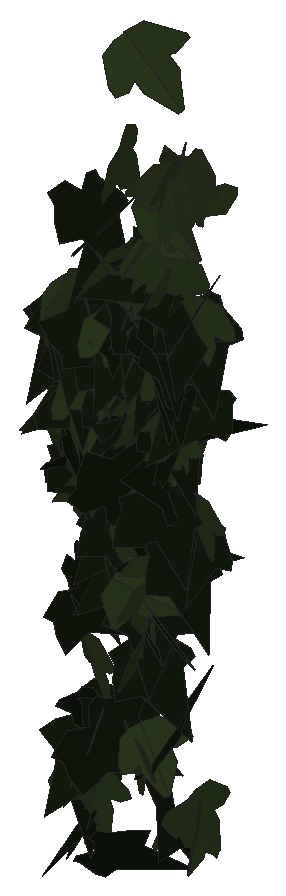
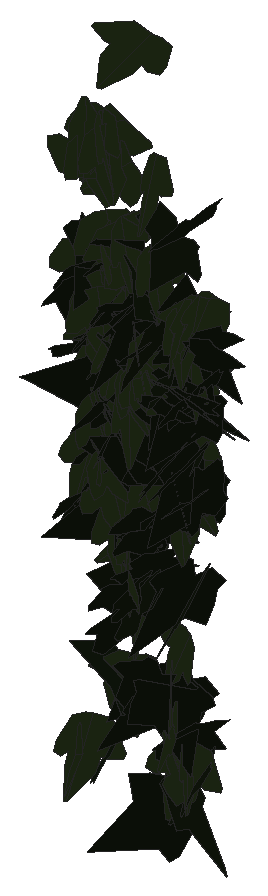
# SketchUp Ruby script. Lengths in inches.
U = 1.inch
M = Sketchup.active_model
def pt(a) = Geom::Point3d.new(a.map { |v| v * U })
def face(e, loops, mat)
  f = e.add_face(loops[0].map { |a| pt(a) })
  loops[1..].each { |l| e.add_face(l.map { |a| pt(a) }).erase! }
  f.material = f.back_material = mat if mat
  f
end
# faces: each face lists its corners as indices into pts; further lists are holes
def faces(e, pts, list, mat = nil) = list.each { |f| face(e, (f[0].is_a?(Array) ? f : [f]).map { |l| l.map { |i| pts[i] } }, mat) }
# xy, xz, yz: faces in a plane at the given z, y or x. An outline is a flat list of corners, or four numbers for a rectangle; further outlines are holes
def ring(l) = l.size == 4 ? [[l[0], l[1]], [l[2], l[1]], [l[2], l[3]], [l[0], l[3]]] : l.each_slice(2).to_a
def flat(e, list, mat, &to3) = list.each { |f| face(e, (f[0].is_a?(Array) ? f : [f]).map { |l| ring(l).map { |u, v| to3.(u, v) } }, mat) }
def xy(e, z, list, mat = nil) = flat(e, list, mat) { |x, y| [x, y, z] }
def xz(e, y, list, mat = nil) = flat(e, list, mat) { |x, z| [x, y, z] }
def yz(e, x, list, mat = nil) = flat(e, list, mat) { |y, z| [x, y, z] }
def lines(e, pts, list) = list.each { |a, b| e.add_line(pt(pts[a]), pt(pts[b])) }
# prism: a flat outline (further loops are holes) pulled along v
def prism(e, loops, v, mat = nil)
  f = face(e, loops, mat); d = Geom::Vector3d.new(v.map { |x| x * U })
  f.pushpull(f.normal.samedirection?(d) ? d.length : -d.length)
end
def box(e, o, s, mat = nil) = prism(e, [[o, [o[0] + s[0], o[1], o[2]], [o[0] + s[0], o[1] + s[1], o[2]], [o[0], o[1] + s[1], o[2]]]], [0, 0, s[2]], mat)
def at(x, y, z, deg = 0) = Geom::Transformation.translation(pt([x, y, z])) * Geom::Transformation.rotation(ORIGIN, Z_AXIS, deg.degrees)
def axes(o, x, y, z) = Geom::Transformation.new([*x, 0, *y, 0, *z, 0, *pt(o).to_a, 1])
def part(name) = M.definitions.add(name)
# library, detail: a bought-in or finely detailed component or shape, given as its bounding box
def library(name, o, s) = part(name).tap { |d| box(d.entities, o, s) }
def detail(e, o, s) = box(e.add_group.entities, o, s)
def put(e, d, t, mat = nil) = e.add_instance(d, t).tap { |i| i.material = mat if mat }
def group(e, t, mat = nil) = e.add_group.tap { |g| g.transformation = t; g.material = mat if mat }.entities
root = M.entities
M.materials.add("efeu1").color = [18, 25, 13]
M.materials.add("efeu2").color = [43, 57, 29]
c1 = part("ivyleaf_9")
p = [[1.54,2.16,1.25],[1.36,2.04,1.19],[-0.21,0.99,0.68],[-0.71,1.11,0.82],[-0.85,0.86,0.67],[-0.8,0.17,0.21],
  [-0.9,-0.01,0.1],[-0.67,-0.16,-0.02],[-0.08,-0.08,-0.05],[-0.03,-0.6,-0.4],[0.65,-0.88,-0.66],[0.83,-0.6,-0.49],
  [1.29,-0.42,-0.43],[1.8125,-0.07,-0.26],[1.21,0.44,0.15]]
faces(c1.entities,p,[[0,1,2,3,4,5,6,7,8,9,10,11,12,13,14]],"efeu1")
c2 = part("ivyleaf_10")
p = [[0,0.5,-0.03],[-0.0625,2.02,-0.43],[-0.19,2.01,-0.46],[-0.54,1.05,-0.29],[-0.52,0.625,-0.18],[-0.83,0.76,-0.28],
  [-1.16,0.64,-0.33],[-1.15,0.33,-0.24],[-0.77,-0.39,0.02],[-0.3,-0.51,0.16],[0.04,-0.48,0.23],[-0.02,2.01,-0.4375],
  [-0.06,2.01,-0.43],[0.04,-0.49,0.23],[0.67,-0.49,0.14],[1.38,0.36,-0.2],[1.375,0.51,-0.24],[0.81,0.65,-0.19],
  [0.62,0.59,-0.15],[0.6,1.09,-0.28],[0.5,1.23,-0.31]]
faces(c2.entities,p,[[0,1,2,3,4,5,6,7,8,9,10],[11,12,0,13,14,15,16,17,18,19,20]],"efeu2")
put(root,c1,axes([533.84,134.95,193.96],[-0.16592,-0.62665,-0.45932],[0.10386,0.44757,-0.64814],[0.76999,-0.19541,-0.01155]))
put(root,c2,axes([533.1,134.63,191.76],[-0.18659,-0.42334,-0.62517],[0.57228,0.34075,-0.40155],[0.49248,-0.55636,0.22975]))
put(root,c2,axes([534.55,135.05,202.51],[-0.46736,-0.64643,0.18683],[-0.07545,-0.17569,-0.79664],[0.66864,-0.47166,0.04069]))
put(root,c2,axes([533.58,134.75,187.75],[0.40332,0.56558,0.24405],[0.1589,0.18631,-0.69437],[-0.59514,0.43303,-0.02001]))
put(root,c1,axes([532.63,134.49,193.875],[-0.1427,-0.17651,0.84402],[0.72497,0.4386,0.2143],[-0.46683,0.73509,0.0748]))
put(root,c2,axes([530.71,135.16,194.8],[-0.30059,0.19641,-0.75857],[0.60278,-0.46117,-0.35826],[-0.50067,-0.67314,0.02411]))
put(root,c2,axes([533.76,134.85,202.09],[0.51875,-0.04959,0.64712],[0.63525,0.20854,-0.49325],[-0.13298,0.80273,0.16812]))
put(root,c2,axes([534.21,134.89,196.51],[-0.68223,-0.41201,-0.00439],[0.00274,0.00396,-0.79699],[0.41203,-0.68223,-0.00197]))
put(root,c1,axes([531.37,134.625,195.06],[0.57411,-0.19969,-0.53388],[-0.46694,0.26982,-0.60305],[0.32691,0.73609,0.07622]))
put(root,c1,axes([533.58,135.35,198.11],[0.13758,-0.75271,0.21451],[0.10161,-0.19877,-0.76268],[0.77605,0.15947,0.06184]))
put(root,c2,axes([533.23,134.77,187.43],[-0.61959,0.35525,0.16784],[-0.16104,0.05627,-0.71356],[-0.35838,-0.63945,0.03046]))
put(root,c2,axes([532.5,134.86,198.36],[0.66095,0.3724,0.21897],[0.16704,0.1488,-0.75726],[-0.3984,0.6802,0.04577]))
put(root,c1,axes([534.33,135.1,192.72],[0.17347,-0.76248,-0.20975],[-0.0096,0.21269,-0.78111],[0.79075,0.16985,0.03653]))
put(root,c1,axes([531.48,135.49,186.59],[-0.39582,-0.61012,0.23934],[-0.07368,-0.2364,-0.7245],[0.65123,-0.39758,0.0635]))
put(root,c1,axes([532.14,134.83,197.82],[-0.63503,-0.42973,0.35723],[0.32377,0.15782,0.76539],[-0.45548,0.71132,0.046]))
put(root,c2,axes([534.24,135.01,203.12],[0.22032,-0.80028,-0.06678],[-0.01386,0.06545,-0.83005],[0.80295,0.22072,0.00399]))
put(root,c2,axes([534.125,135.05,200.32],[-0.64051,-0.45772,0.15302],[-0.09081,-0.13544,-0.78522],[0.474,-0.64445,0.05634]))
put(root,c1,axes([531.2,135.29,197.93],[-0.75961,-0.27683,-0.11932],[0.10828,0.05132,-0.8084],[0.28133,-0.76721,-0.01102]))
put(root,c2,axes([531.57,134.96,196.35],[0.34137,0.71991,-0.0217],[-0.00719,-0.02061,-0.79674],[-0.7202,0.34144,-0.00234]))
put(root,c1,axes([533.98,135.39,197.95],[0.13306,-0.79394,0.12439],[-0.00172,-0.12636,-0.8047],[0.80362,0.13118,-0.02231]))
put(root,c1,axes([532.14,135.25,196.45],[-0.81999,-0.00074,0.27979],[-0.27979,0.00771,-0.81995],[-0.00179,-0.86637,-0.00754]))
put(root,c2,axes([533.41,134.98,191.61],[0.03767,-0.74397,-0.14396],[-0.0036,0.14396,-0.74491],[0.75776,0.03767,0.00362]))
put(root,c2,axes([533.67,135.02,199.05],[-0.80206,-0.11083,0.10074],[-0.08251,-0.13107,-0.80109],[0.125,-0.79766,0.11763]))
put(root,c1,axes([531.24,135.35,198.1],[-0.31647,-0.71563,-0.13253],[0.05105,0.12233,-0.78248],[0.72601,-0.32055,-0.00274]))
put(root,c2,axes([533.07,135,199.59],[-0.6543,-0.46309,0.03838],[-0.03555,-0.0162,-0.80156],[0.46331,-0.65522,-0.0073]))
put(root,c2,axes([531.23,134.66,198.75],[-0.04867,-0.59501,-0.55283],[0.24229,0.51797,-0.57882],[0.77521,-0.19924,0.1462]))
put(root,c1,axes([533.71,135.63,194.3125],[-0.2466,-0.13898,0.76089],[-0.18699,-0.76422,-0.2002],[0.75053,-0.23607,0.20012]))
put(root,c1,axes([534.69,135.6,197.02],[-0.52563,-0.56705,0.21694],[-0.02156,-0.26933,-0.75623],[0.60674,-0.50081,0.16106]))
put(root,c1,axes([532.72,135.4,198.29],[-0.64504,-0.46675,-0.16169],[0.15465,0.06176,-0.79521],[0.46914,-0.66212,0.03981]))
put(root,c1,axes([533.83,135.49,200.02],[-0.69769,-0.06374,0.38908],[-0.33584,-0.31818,-0.65436],[0.20653,-0.73274,0.25029]))
put(root,c2,axes([533.9,135.25,199.98],[0.2862,-0.75883,0.13365],[0.07281,-0.11529,-0.81055],[0.76706,0.29407,0.02708]))
put(root,c1,axes([534.41,135.47,199.37],[-0.18346,-0.78927,0.02669],[-0.00748,-0.02566,-0.81031],[0.78968,-0.18361,-0.00147]))
put(root,c1,axes([533.71,135.5,198.39],[0.17171,-0.75603,0.22366],[0.04403,-0.21935,-0.77527],[0.78719,0.17718,-0.00542]))
put(root,c1,axes([531.46,135.08,201.39],[0.31522,-0.69824,-0.32345],[0.00014,0.34959,-0.75452],[0.76952,0.28596,0.13264]))
put(root,c2,axes([534.05,135.14,202.87],[-0.32805,-0.75834,0.01412],[-0.00416,-0.01359,-0.82625],[0.75846,-0.32808,0.00158]))
put(root,c1,axes([533.875,135.48,198.03],[-0.6926,-0.32698,-0.26214],[0.30707,-0.05135,-0.74726],[0.2852,-0.73876,0.16797]))
put(root,c1,axes([531,135.54,185.22],[0.19734,-0.60262,0.41738],[0.13128,-0.3962,-0.63411],[0.72119,0.23702,0.00122]))
put(root,c1,axes([532.15,134.57,187.58],[0.1151,-0.15435,-0.89731],[-0.02892,0.90337,-0.1591],[0.91002,0.04823,0.10843]))
put(root,c2,axes([533.03,135.11,193.22],[-0.68755,-0.05511,0.38302],[-0.37043,-0.1321,-0.68395],[0.11191,-0.77587,0.08924]))
put(root,c1,axes([533.79,135.2,197.21],[-0.66198,0.42777,-0.04278],[-0.04593,-0.14846,-0.77388],[-0.42745,-0.64653,0.14939]))
put(root,c2,axes([531.19,134.84,198.81],[0.36313,0.65044,0.29531],[0.03551,0.31443,-0.73622],[-0.71346,0.34671,0.11366]))
put(root,c2,axes([532.39,135.41,196.875],[-0.22167,-0.71925,0.27722],[0.08408,-0.3093,-0.73524],[0.76623,-0.17414,0.16088]))
put(root,c2,axes([531.83,134.96,196.71],[-0.60272,0.50627,0.13738],[-0.12829,0.06065,-0.78634],[-0.50865,-0.6152,0.03553]))
put(root,c1,axes([533.62,135.73,185.44],[0.03368,-0.50018,0.60049],[0.05559,-0.59799,-0.50122],[0.77954,0.06425,0.0098]))
put(root,c2,axes([531.52,135.06,196.86],[-0.72153,0.24589,0.17205],[-0.19184,-0.03337,-0.75681],[-0.23078,-0.74101,0.09117]))
put(root,c2,axes([534.47,135.04,203.21],[-0.79112,0.17971,-0.03596],[0.03633,-0.00237,-0.81125],[-0.17963,-0.79193,-0.00573]))
put(root,c2,axes([533.54,135.26,200.47],[0.39155,0.66223,-0.25685],[-0.22739,-0.16099,-0.76171],[-0.67291,0.43973,0.10795]))
put(root,c2,axes([531.54,135.07,185.85],[-0.83355,-0.12212,-0.11742],[0.11619,0.01695,-0.84245],[0.12329,-0.84161,0.00007]))
put(root,c1,axes([531.68,135.18,184.96],[-0.58553,0.59707,-0.21516],[0.14057,-0.16346,-0.83615],[-0.61889,-0.60202,0.01364]))
put(root,c2,axes([533.13,134.91,205.9375],[0.52377,0.47337,0.55455],[0.40242,0.3817,-0.70591],[-0.608,0.66043,0.0105]))
put(root,c2,axes([533.1875,134.99,189.97],[0.15695,-0.66236,-0.39426],[-0.07468,0.3874,-0.68055],[0.7672,0.17321,0.01441]))
put(root,c1,axes([531.59,135.59,196.4375],[-0.76138,-0.19307,0.15907],[-0.13583,-0.10885,-0.78229],[0.21007,-0.77017,0.07069]))
put(root,c1,axes([533.46,135.69,197.37],[0.13564,-0.70848,0.34338],[0.07348,-0.33552,-0.7213],[0.78387,0.15404,0.0082]))
put(root,c1,axes([531.65,134.91,197.01],[0.69236,0.31292,-0.17973],[-0.1589,-0.08477,-0.7597],[-0.324,0.71027,-0.01149]))
put(root,c1,axes([533.12,135.625,198.68],[-0.34448,-0.72407,-0.02238],[0.01031,0.01988,-0.80183],[0.72434,-0.34463,0.00077]))
put(root,c2,axes([534.65,135.35,202.18],[-0.64248,-0.49641,-0.04392],[-0.03738,-0.02344,0.8119],[-0.49695,0.64355,-0.0043]))
put(root,c1,axes([533.93,135.34,195.5625],[-0.68086,0.33892,-0.24015],[0.21236,-0.11228,-0.76053],[-0.35699,-0.71319,0.00561]))
put(root,c1,axes([530.98,135.6,196.75],[0.03615,-0.7984,0.06051],[0.00888,-0.06017,-0.7992],[0.80064,0.03672,0.00613]))
put(root,c2,axes([533.51,135.2,192.21],[-0.39062,-0.68014,-0.06591],[0.027,0.06049,-0.7843],[0.68279,-0.3915,-0.00669]))
put(root,c1,axes([532.9,135.35,198.59],[0.28315,-0.72603,-0.20516],[-0.03004,0.2081,-0.77793],[0.75386,0.28099,0.04605]))
put(root,c2,axes([532.28,135.42,197.72],[-0.42013,-0.63714,0.21631],[-0.06227,-0.2171,-0.76042],[0.66997,-0.41972,0.06496]))
put(root,c2,axes([534.72,135.28,199.36],[-0.81575,-0.02654,-0.01615],[0.02151,-0.17598,-0.79686],[0.02242,-0.79671,0.17655]))
put(root,c2,axes([532.41,135.3,200.01],[-0.02902,-0.81791,-0.02892],[0.00048,0.02892,-0.81843],[0.81842,-0.02902,-0.00054]))
put(root,c1,axes([532.15,135.25,197.62],[0.11647,-0.66884,-0.43019],[0.10154,0.44373,-0.6624],[0.78873,0.04164,0.1488]))
put(root,c2,axes([534.01,135.28,198.74],[-0.59541,-0.53303,0.03518],[-0.00742,-0.04443,-0.79865],[0.53413,-0.59479,0.02813]))
put(root,c2,axes([531.4,135.18,186.09],[0.18111,-0.70138,-0.23666],[0.00765,0.2454,-0.72143],[0.74019,0.16907,0.06536]))
put(root,c1,axes([533.87,134.74,187.29],[-0.42501,0.76807,-0.09642],[-0.05251,0.08114,0.87779],[0.77231,0.42819,0.00662]))
put(root,c2,axes([533.65,135.62,193.99],[-0.20431,-0.64905,0.38443],[-0.03336,-0.39011,-0.67638],[0.75361,-0.19323,0.07427]))
put(root,c1,axes([534.84,134.65,199.16],[-0.0015,0.58299,0.5786],[0.00072,0.5786,-0.58299],[-0.82137,-0.00056,-0.00157]))
put(root,c2,axes([531.52,135.29,189.25],[-0.60517,0.36773,-0.23142],[0.17428,-0.15802,-0.70687],[-0.398,-0.62835,0.04233]))
put(root,c2,axes([533.02,135.51,196.48],[0.04216,-0.76807,0.17268],[-0.00077,-0.17297,-0.76916],[0.78724,0.04097,-0.01]))
put(root,c2,axes([534.0625,135.17,197.68],[0.3737,0.69499,0.06481],[-0.08724,0.11944,-0.77781],[-0.69253,0.35998,0.13295]))
put(root,c2,axes([533.73,135.42,193.22],[-0.52883,-0.53696,0.20001],[-0.1249,-0.15761,-0.75336],[0.55922,-0.54298,0.02089]))
put(root,c2,axes([531.47,135.04,193.67],[0.29315,-0.06457,-0.73666],[-0.58044,0.47088,-0.27226],[0.45817,0.63786,0.12641]))
put(root,c2,axes([532.92,135.3125,197.77],[0.33957,-0.71193,-0.17092],[-0.04585,0.16736,-0.7882],[0.73072,0.34134,0.02997]))
put(root,c1,axes([532.73,135.6,190.74],[0.49296,-0.46005,0.45299],[0.32039,-0.32051,-0.67415],[0.56053,0.58778,-0.01306]))
put(root,c1,axes([531.54,134.875,190.9375],[0.0862,-0.2132,-0.83177],[-0.22329,0.80162,-0.22862],[0.82912,0.23805,0.02491]))
put(root,c2,axes([533.27,135.41,200.59],[0.08287,-0.79862,-0.0637],[-0.00316,0.06371,-0.8029],[0.80115,0.08286,0.00342]))
put(root,c1,axes([531.53,135.67,197.35],[0.43106,-0.60047,0.29196],[0.15014,-0.25145,-0.73882],[0.65059,0.45588,-0.02294]))
put(root,c1,axes([531.18,135,196.37],[0.68529,0.36969,0.0047],[0.00342,0.00355,-0.77865],[-0.3697,0.6853,0.0015]))
put(root,c2,axes([533.58,135.31,197.13],[-0.14292,-0.74798,-0.20845],[0.20713,0.16754,-0.74322],[0.74834,-0.18923,0.16591]))
put(root,c1,axes([533.13,135.375,189.61],[0.13694,-0.65932,-0.42332],[0.05373,0.43662,-0.66267],[0.78167,0.08549,0.11971]))
put(root,c1,axes([534.48,135.6,198.93],[-0.0165,-0.76827,-0.23708],[0.01297,0.23685,-0.76841],[0.80391,-0.01958,0.00753]))
put(root,c2,axes([531.99,135.04,187.86],[0.12348,-0.41131,-0.65224],[-0.21939,0.61451,-0.42905],[0.73923,0.25108,-0.01838]))
put(root,c1,axes([531.82,135.375,187.84],[0.31205,0.47796,-0.50456],[-0.27493,-0.42307,-0.57081],[-0.63831,0.41588,-0.00081]))
put(root,c2,axes([531.45,135.4375,198.62],[0.01819,-0.80368,-0.13874],[0.029,0.13933,-0.80326],[0.81505,0.01298,0.03168]))
put(root,c1,axes([532.03,134.83,200.65],[0.18016,0.59753,0.49537],[-0.06744,0.51866,-0.6011],[-0.77323,0.09399,0.16785]))
put(root,c1,axes([532.02,134.97,184.09],[0.63363,0.29881,0.43485],[0.37735,0.21833,-0.69986],[-0.36877,0.73683,0.03103]))
put(root,c1,axes([531.5625,135.78,196.79],[-0.78567,0.00982,-0.0405],[0.03825,-0.13325,-0.77446],[-0.01652,-0.77534,0.13259]))
put(root,c1,axes([534.22,135.96,193],[-0.1481,-0.73998,0.15713],[0.00431,-0.16094,-0.75384],[0.75647,-0.14395,0.03506]))
put(root,c1,axes([532.26,135.56,192.86],[-0.12798,-0.65228,-0.39742],[0.05354,0.39431,-0.66441],[0.76194,-0.13728,-0.02007]))
put(root,c2,axes([532.33,135.74,196.99],[-0.4182,-0.61769,0.25766],[0.01408,-0.31188,-0.72482],[0.66913,-0.37949,0.17629]))
put(root,c1,axes([532.95,134.93,198.94],[-0.52428,0.35493,-0.59809],[-0.51385,0.30705,0.63265],[0.46866,0.7337,0.02457]))
put(root,c1,axes([532.96,135.81,190.68],[-0.16209,-0.7336,-0.13136],[0.00844,0.13261,-0.75103],[0.74522,-0.16107,-0.02006]))
put(root,c1,axes([533.38,134.88,192.48],[0.0592,0.32601,-0.80092],[0.07117,0.79824,0.33018],[0.8618,-0.08832,0.02775]))
put(root,c1,axes([530.47,135.86,193.76],[0.05316,-0.32791,0.71492],[0.51605,-0.52622,-0.27974],[0.59358,0.48686,0.17917]))
put(root,c2,axes([531.44,135.59,194.02],[0.41017,-0.64712,-0.09094],[-0.05793,0.07093,-0.76609],[0.65091,0.4141,-0.01088]))
put(root,c2,axes([531.4,135.53,185.39],[0.37193,-0.67752,0.04244],[-0.00023,0.04827,0.77255],[-0.67885,-0.37121,0.023]))
put(root,c1,axes([533.73,135.18,195.9],[0.48806,-0.02782,0.67419],[0.65889,0.19906,-0.46877],[-0.1455,0.80815,0.13867]))
put(root,c1,axes([532.37,136.12,191.53],[-0.47989,-0.4714,0.36402],[-0.15741,-0.35048,-0.66137],[0.57441,-0.48987,0.12289]))
put(root,c1,axes([532.28,135.87,196.1875],[-0.72832,-0.28605,-0.10521],[0.10288,0.02582,-0.78237],[0.2869,-0.73543,0.01345]))
put(root,c1,axes([532.13,136.08,192.71],[-0.47698,-0.5663,0.23462],[-0.10824,-0.2148,-0.73851],[0.60335,-0.48623,0.05299]))
put(root,c2,axes([534.34,136.03,185.45],[-0.07142,0.40787,-0.73489],[0.12034,-0.72497,-0.41406],[-0.83182,-0.1399,0.00319]))
put(root,c1,axes([531.55,135.67,194.75],[0.33761,-0.68678,-0.13482],[-0.02899,0.13583,-0.76454],[0.69928,0.3372,0.03339]))
put(root,c2,axes([533.95,135.77,195.4],[-0.10936,-0.76234,0.19115],[0.01716,-0.19527,-0.76892],[0.78576,-0.10183,0.0434]))
put(root,c1,axes([532.29,135.99,190.24],[0.22448,-0.51028,0.52232],[0.28366,-0.44259,-0.5543],[0.67287,0.35682,0.05942]))
put(root,c1,axes([530.875,135.8,193.8125],[0.13884,-0.74851,-0.12847],[0.11793,0.15027,-0.74803],[0.75024,0.1149,0.14136]))
put(root,c2,axes([533.61,135.67,195.51],[0.74811,-0.06392,0.21382],[0.21656,0.02721,-0.74956],[0.05392,0.77759,0.0438]))
put(root,c1,axes([532.08,135.5,188.21],[-0.11314,-0.32849,-0.69932],[0.38646,0.58795,-0.3387],[0.66903,-0.39517,0.07738]))
put(root,c1,axes([532.2,135.3125,198.71],[0.70697,0.02914,-0.36758],[-0.36854,0.08141,-0.70237],[0.01186,0.79265,0.08565]))
put(root,c1,axes([533.5,135.82,195.83],[0.16617,-0.76108,-0.1501],[-0.00411,0.15264,-0.77851],[0.77573,0.16384,0.02803]))
put(root,c2,axes([533.87,135.73,198.48],[-0.55071,-0.56145,0.13126],[-0.03853,-0.14527,-0.78303],[0.5753,-0.54718,0.07321]))
put(root,c2,axes([531.36,135.92,187.15],[-0.17333,0.57007,-0.49948],[0.05388,-0.50181,-0.59143],[-0.75602,-0.16646,0.07237]))
put(root,c1,axes([533.8,135.71,193.98],[-0.50523,0.11969,0.6047],[-0.58629,0.14819,-0.51918],[-0.19039,-0.77392,-0.00589]))
put(root,c2,axes([532.35,135.36,202.68],[0.12007,-0.66211,-0.46399],[0.05262,0.47448,-0.66347],[0.80678,0.06759,0.11233]))
put(root,c1,axes([530.91,135.55,191.09],[0.50601,-0.45467,-0.35821],[-0.26929,0.23625,-0.68026],[0.51237,0.57319,-0.00376]))
put(root,c2,axes([531.25,135.7,193.55],[-0.18863,-0.74442,-0.03497],[0.02005,0.03099,-0.76785],[0.74497,-0.18932,0.01181]))
put(root,c1,axes([531.02,135.93,194.77],[0.2189,-0.75711,-0.01729],[0.03612,0.02842,-0.78697],[0.75645,0.21773,0.04258]))
put(root,c1,axes([532.75,135.23,198.25],[0.10892,-0.2256,-0.76858],[-0.28046,0.71581,-0.24985],[0.7503,0.30032,0.01817]))
put(root,c2,axes([534.41,135.59,193.97],[-0.72361,0.2994,-0.01837],[0.01333,-0.01582,-0.78304],[-0.29966,-0.72367,0.00952]))
put(root,c2,axes([532.6,136.01,191.18],[0.38623,-0.32482,0.60183],[0.54425,-0.27254,-0.49638],[0.41412,0.66113,0.09106]))
put(root,c1,axes([532.03,136.09,192.73],[-0.19168,-0.75307,-0.01706],[0.00546,0.01621,-0.77708],[0.75325,-0.19175,0.00129]))
put(root,c2,axes([532.92,135.65,195.875],[-0.01768,-0.77943,-0.18772],[-0.0028,0.18783,-0.7796],[0.80172,-0.01654,-0.00687]))
put(root,c2,axes([531.41,135.36,198.87],[-0.33234,0.59061,0.40272],[-0.23383,0.32986,-0.67673],[-0.67552,-0.40475,0.03612]))
put(root,c1,axes([531.01,135.12,194.28],[0.38369,0.6771,0.32218],[0.16208,0.27846,-0.77825],[-0.73211,0.41651,-0.00345]))
put(root,c2,axes([534.35,135.51,185.83],[-0.28325,-0.75644,-0.39193],[0.18087,0.35022,-0.80664],[0.83252,-0.33344,0.0419]))
